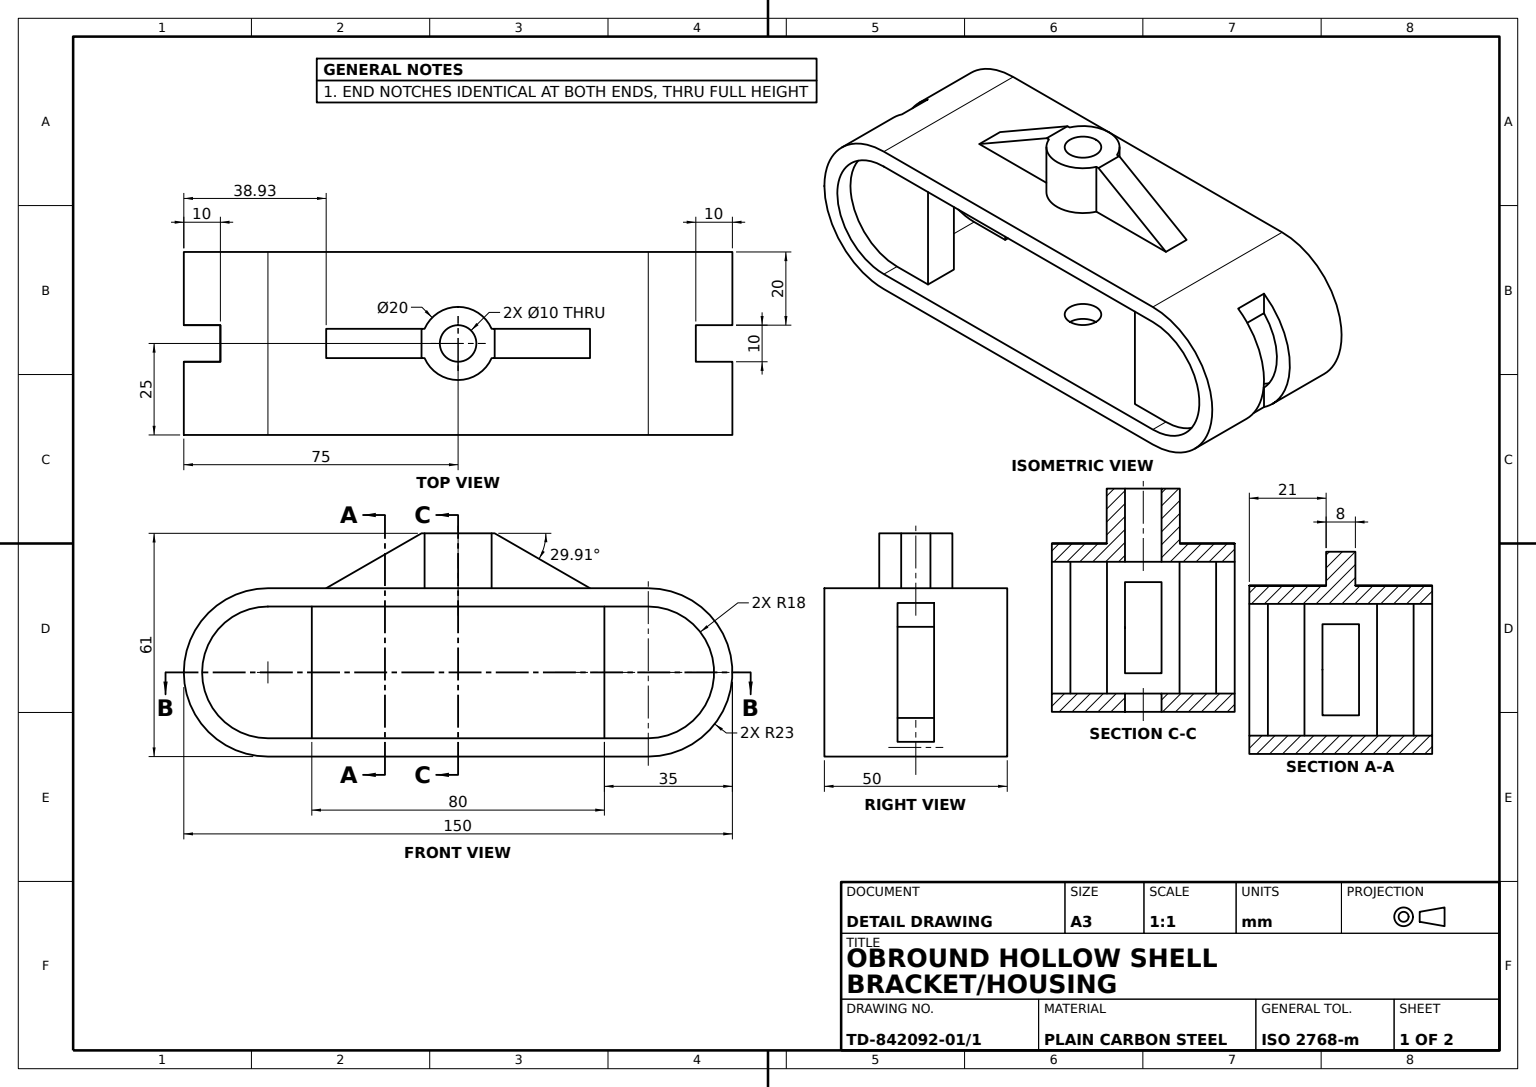
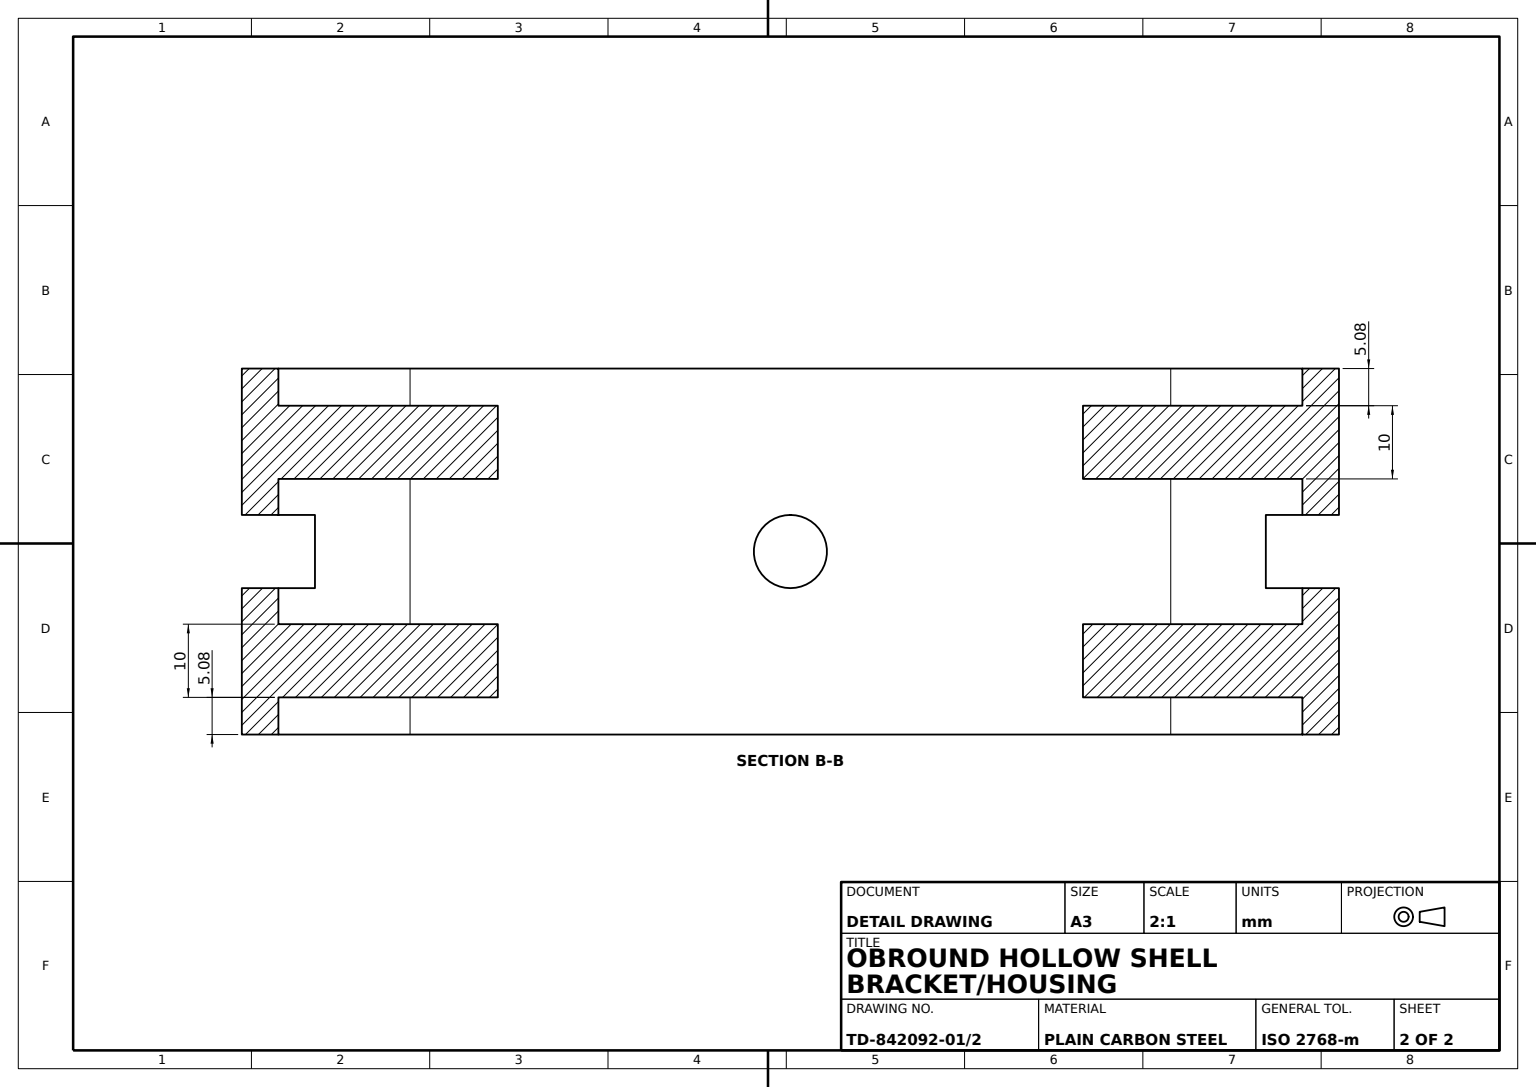
solid
v1 (-52,-18,25)
v2 (-52,-18,19.922192)
e1 v1 v2 LINE
v3 (-70,0,19.922192)
e2 v2 v3 CIRCLE(AX(P(-52,0,19.922192),D(0,0,-1),D(1,0,0)),18)
v4 (-70,0,25)
e3 v4 v3 LINE
e4 v4 v1 CIRCLE(AX(P(-52,0,25),D(0,0,1),D(1,0,0)),18)
face CYL(AX(P(-52,0,25),D(0,0,-1),D(-1,0,0)),18) rev [e1 e2 -e3 e4]
v5 (0,-23,-5)
v6 (0,-23,5)
e5 v5 v6 CIRCLE(AX(P(0,-23,0),D(0,1,0),D(0,0,1)),5)
v7 (0,-18,-5)
e6 v5 v7 LINE
v8 (0,-18,5)
e7 v7 v8 CIRCLE(AX(P(0,-18,0),D(0,1,0),D(-1,0,0)),5)
e8 v6 v8 LINE
face CYL(AX(P(0,-27,0),D(0,1,0),D(0,0,1)),5) rev [-e5 e6 e7 -e8]
v9 (40,-18,-19.922192)
v10 (40,18,-19.922192)
e9 v9 v10 LINE
v11 (40,-18,-9.922192)
e10 v11 v9 LINE
v12 (40,18,-9.922192)
e11 v11 v12 LINE
e12 v10 v12 LINE
face PLANE(AX(P(40,-23.002,-19.922192),D(-1,0,0),D(0,-1,0))) [-e9 -e10 e11 -e12]
e13 v6 v5 CIRCLE(AX(P(0,-23,0),D(0,1,0),D(0,0,1)),5)
v13 (-52,-23,25)
v14 (-52,-23,-25)
e14 v13 v14 LINE
v15 (52,-23,-25)
e15 v14 v15 LINE
v16 (52,-23,25)
e16 v16 v15 LINE
e17 v13 v16 LINE
face PLANE(AX(P(-52,-23,25),D(0,1,0),D(0,0,1))) rev [e13 e5] [e14 e15 -e16 -e17]
v17 (65,-18.973666,-5)
v18 (65,-12.4499,-5)
e18 v17 v18 LINE
v19 (65,-12.4499,5)
e19 v18 v19 LINE
v20 (65,-18.973666,5)
e20 v20 v19 LINE
e21 v17 v20 LINE
face PLANE(AX(P(65,-27,-5),D(-1,0,0),D(0,0,1))) rev [e18 e19 -e20 -e21]
v21 (-52,18,-19.922192)
v22 (-52,18,-25)
e22 v21 v22 LINE
v23 (-70,0,-19.922192)
e23 v23 v21 CIRCLE(AX(P(-52,0,-19.922192),D(0,0,-1),D(1,0,0)),18)
v24 (-70,0,-25)
e24 v23 v24 LINE
e25 v22 v24 CIRCLE(AX(P(-52,0,-25),D(0,0,1),D(1,0,0)),18)
face CYL(AX(P(-52,0,25),D(0,0,-1),D(-1,0,0)),18) rev [-e22 -e23 e24 -e25]
v25 (-10,38,4)
v26 (-36.072943,23,4)
e26 v25 v26 LINE
v27 (-9.165151,23,4)
e27 v27 v26 LINE
v28 (-9.165151,38,4)
e28 v28 v27 LINE
e29 v28 v25 LINE
face PLANE(AX(P(0,7.5,4),D(0,0,1),D(1,0,0))) [e26 -e27 -e28 e29]
v29 (-65,18.973666,-5)
v30 (-65,18.973666,5)
e30 v29 v30 LINE
v31 (-75,0,5)
e31 v30 v31 CIRCLE(AX(P(-52,0,5),D(0,0,1),D(1,0,0)),23)
v32 (-75,0,25)
e32 v32 v31 LINE
v33 (-52,23,25)
e33 v33 v32 CIRCLE(AX(P(-52,0,25),D(0,0,1),D(1,0,0)),23)
v34 (-52,23,-25)
e34 v33 v34 LINE
v35 (-75,0,-25)
e35 v34 v35 CIRCLE(AX(P(-52,0,-25),D(0,0,1),D(1,0,0)),23)
v36 (-75,0,-5)
e36 v36 v35 LINE
e37 v36 v29 CIRCLE(AX(P(-52,0,-5),D(0,0,-1),D(-1,0,0)),23)
face CYL(AX(P(-52,0,25),D(0,0,-1),D(-1,0,0)),23) [e30 e31 -e32 -e33 e34 e35 -e36 e37]
v37 (-65,12.4499,5)
v38 (-70,0,5)
e38 v37 v38 CIRCLE(AX(P(-52,0,5),D(0,0,1),D(1,0,0)),18)
v39 (-65,12.4499,-5)
e39 v39 v37 LINE
v40 (-70,0,-5)
e40 v40 v39 CIRCLE(AX(P(-52,0,-5),D(0,0,-1),D(-1,0,0)),18)
v41 (-70,0,-9.922192)
e41 v40 v41 LINE
v42 (-52,18,-9.922192)
e42 v42 v41 CIRCLE(AX(P(-52,0,-9.922192),D(0,0,1),D(-1,0,0)),18)
v43 (-52,18,9.922192)
e43 v43 v42 LINE
v44 (-70,0,9.922192)
e44 v43 v44 CIRCLE(AX(P(-52,0,9.922192),D(0,0,1),D(-1,0,0)),18)
e45 v44 v38 LINE
face CYL(AX(P(-52,0,25),D(0,0,-1),D(-1,0,0)),18) rev [-e38 -e39 -e40 e41 -e42 -e43 e44 e45]
v45 (-40,-18,-9.922192)
v46 (-40,18,-9.922192)
e46 v45 v46 LINE
e47 v46 v42 LINE
v47 (-52,-18,-9.922192)
e48 v41 v47 CIRCLE(AX(P(-52,0,-9.922192),D(0,0,1),D(-1,0,0)),18)
e49 v47 v45 LINE
face PLANE(AX(P(-40,-23.002,-9.922192),D(0,0,-1),D(-1,0,0))) rev [e46 e47 e42 e48 e49]
v48 (-52,-18,-19.922192)
e50 v48 v23 CIRCLE(AX(P(-52,0,-19.922192),D(0,0,-1),D(1,0,0)),18)
v49 (-52,-18,-25)
e51 v48 v49 LINE
e52 v24 v49 CIRCLE(AX(P(-52,0,-25),D(0,0,1),D(1,0,0)),18)
face CYL(AX(P(-52,0,25),D(0,0,-1),D(-1,0,0)),18) rev [-e24 -e50 e51 -e52]
v50 (52,23,-25)
e53 v50 v34 LINE
v51 (52,23,25)
e54 v51 v33 LINE
e55 v51 v50 LINE
v52 (36.072943,23,-4)
v53 (36.072943,23,4)
e56 v52 v53 LINE
v54 (9.165151,23,4)
e57 v53 v54 LINE
e58 v27 v54 CIRCLE(AX(P(0,23,0),D(0,1,0),D(0,0,-1)),10)
v55 (-36.072943,23,-4)
e59 v26 v55 LINE
v56 (-9.165151,23,-4)
e60 v56 v55 LINE
v57 (0,23,-10)
e61 v57 v56 CIRCLE(AX(P(0,23,0),D(0,1,0),D(0,0,-1)),10)
v58 (9.165151,23,-4)
e62 v58 v57 CIRCLE(AX(P(0,23,0),D(0,1,0),D(0,0,-1)),10)
e63 v52 v58 LINE
face PLANE(AX(P(-52,23,25),D(0,-1,0),D(0,0,-1))) rev [e53 -e34 -e54 e55] [e56 e57 -e58 e27 e59 -e60 -e61 -e62 -e63]
v59 (10,38,-4)
v60 (10,38,4)
e64 v59 v60 LINE
e65 v60 v53 LINE
e66 v59 v52 LINE
face PLANE(AX(P(10,38,0),D(-0.498672433,-0.866790519,0),D(0.866790519,-0.498672433,0))) rev [e64 e65 -e56 -e66]
v61 (-65,-12.4499,5)
v62 (-65,-12.4499,-5)
e67 v61 v62 LINE
e68 v38 v61 CIRCLE(AX(P(-52,0,5),D(0,0,1),D(1,0,0)),18)
v63 (-52,-18,9.922192)
e69 v44 v63 CIRCLE(AX(P(-52,0,9.922192),D(0,0,1),D(-1,0,0)),18)
e70 v63 v47 LINE
e71 v62 v40 CIRCLE(AX(P(-52,0,-5),D(0,0,-1),D(-1,0,0)),18)
face CYL(AX(P(-52,0,25),D(0,0,-1),D(-1,0,0)),18) rev [-e67 -e68 -e45 e69 e70 -e48 -e41 -e71]
e72 v8 v7 CIRCLE(AX(P(0,-18,0),D(0,1,0),D(-1,0,0)),5)
face CYL(AX(P(0,-27,0),D(0,1,0),D(0,0,1)),5) rev [e72 -e6 -e13 e8]
v64 (0,38,5)
v65 (0,38,-5)
e73 v64 v65 CIRCLE(AX(P(0,38,0),D(0,1,0),D(0,0,1)),5)
e74 v65 v64 CIRCLE(AX(P(0,38,0),D(0,1,0),D(0,0,1)),5)
v66 (-9.165151,38,-4)
v67 (-10,38,-4)
e75 v66 v67 LINE
e76 v67 v25 LINE
v68 (9.165151,38,4)
e77 v28 v68 CIRCLE(AX(P(0,38,0),D(0,1,0),D(0,0,1)),10)
e78 v68 v60 LINE
v69 (9.165151,38,-4)
e79 v69 v59 LINE
v70 (0,38,-10)
e80 v69 v70 CIRCLE(AX(P(0,38,0),D(0,1,0),D(0,0,1)),10)
e81 v70 v66 CIRCLE(AX(P(0,38,0),D(0,1,0),D(0,0,1)),10)
face PLANE(AX(P(0,38,0),D(0,1,0),D(0,0,1))) [-e73 -e74] [e75 e76 -e29 e77 e78 -e64 -e79 e80 e81]
v71 (40,-18,9.922192)
v72 (40,18,9.922192)
e82 v71 v72 LINE
v73 (40,-18,19.922192)
e83 v71 v73 LINE
v74 (40,18,19.922192)
e84 v73 v74 LINE
e85 v74 v72 LINE
face PLANE(AX(P(40,-23.002,19.922192),D(1,0,0),D(0,1,0))) rev [-e82 e83 e84 e85]
v75 (-40,-18,-19.922192)
e86 v75 v48 LINE
v76 (-40,18,-19.922192)
e87 v21 v76 LINE
e88 v75 v76 LINE
face PLANE(AX(P(-70,-23.002,-19.922192),D(0,0,1),D(1,0,0))) rev [e86 e50 e23 e87 -e88]
e89 v39 v29 LINE
v77 (-65,-18.973666,-5)
e90 v77 v36 CIRCLE(AX(P(-52,0,-5),D(0,0,-1),D(-1,0,0)),23)
e91 v77 v62 LINE
face PLANE(AX(P(-65,-27,-5),D(0,0,-1),D(-1,0,0))) rev [e89 -e37 -e90 e91 e71 e40]
v78 (65,18.973666,5)
e92 v20 v78 CIRCLE(AX(P(52,0,5),D(0,0,1),D(1,0,0)),23)
v79 (65,12.4499,5)
e93 v19 v79 CIRCLE(AX(P(52,0,5),D(0,0,1),D(1,0,0)),18)
e94 v79 v78 LINE
face PLANE(AX(P(65,-27,5),D(0,0,1),D(1,0,0))) rev [-e92 e20 e93 e94]
e95 v66 v56 LINE
e96 v70 v57 LINE
face CYL(AX(P(0,38,0),D(0,-1,0),D(0,0,-1)),10) [-e95 -e81 e96 e61]
e97 v67 v55 LINE
face PLANE(AX(P(-10,38,0),D(-0.498672433,0.866790519,0),D(-0.866790519,-0.498672433,0))) [-e76 e97 -e59 -e26]
v80 (52,18,9.922192)
e98 v72 v80 LINE
v81 (52,-18,9.922192)
e99 v80 v81 CIRCLE(AX(P(52,0,9.922192),D(0,0,-1),D(1,0,0)),18)
e100 v81 v71 LINE
face PLANE(AX(P(40,-23.002,9.922192),D(0,0,1),D(1,0,0))) rev [e82 e98 e99 e100]
v82 (-65,-18.973666,5)
e101 v82 v77 LINE
e102 v82 v61 LINE
face PLANE(AX(P(-65,-27,5),D(1,0,0),D(0,0,-1))) rev [-e91 -e101 e102 e67]
e103 v54 v68 LINE
face PLANE(AX(P(0,7.5,4),D(0,0,1),D(1,0,0))) [-e78 -e103 -e57 -e65]
face CYL(AX(P(0,38,0),D(0,-1,0),D(0,0,-1)),10) [e28 e58 e103 -e77]
e104 v35 v14 CIRCLE(AX(P(-52,0,-25),D(0,0,1),D(1,0,0)),23)
e105 v32 v13 CIRCLE(AX(P(-52,0,25),D(0,0,1),D(1,0,0)),23)
e106 v31 v82 CIRCLE(AX(P(-52,0,5),D(0,0,1),D(1,0,0)),23)
face CYL(AX(P(-52,0,25),D(0,0,-1),D(-1,0,0)),23) [e101 e90 e36 e104 -e14 -e105 e32 e106]
v83 (-40,-18,19.922192)
v84 (-40,18,19.922192)
e107 v83 v84 LINE
v85 (-52,18,19.922192)
e108 v85 v84 LINE
e109 v3 v85 CIRCLE(AX(P(-52,0,19.922192),D(0,0,-1),D(1,0,0)),18)
e110 v83 v2 LINE
face PLANE(AX(P(-70,-23.002,19.922192),D(0,0,1),D(1,0,0))) [e107 -e108 -e109 -e2 -e110]
v86 (52,18,-9.922192)
e111 v12 v86 LINE
e112 v80 v86 LINE
v87 (52,18,19.922192)
e113 v87 v74 LINE
v88 (52,18,25)
e114 v88 v87 LINE
v89 (-52,18,25)
e115 v88 v89 LINE
e116 v89 v85 LINE
v90 (-40,18,9.922192)
e117 v84 v90 LINE
e118 v90 v43 LINE
e119 v76 v46 LINE
v91 (52,18,-25)
e120 v91 v22 LINE
v92 (52,18,-19.922192)
e121 v92 v91 LINE
e122 v92 v10 LINE
v93 (0,18,-5)
v94 (0,18,5)
e123 v93 v94 CIRCLE(AX(P(0,18,0),D(0,-1,0),D(1,0,0)),5)
e124 v94 v93 CIRCLE(AX(P(0,18,0),D(0,-1,0),D(1,0,0)),5)
face PLANE(AX(P(-52,18,25),D(0,-1,0),D(1,0,0))) [e111 -e112 -e98 -e85 -e113 -e114 e115 e116 e108 e117 e118 e43 -e47 -e119 -e87 e22 -e120 -e121 e122 e12] [-e123 -e124]
e125 v89 v4 CIRCLE(AX(P(-52,0,25),D(0,0,1),D(1,0,0)),18)
face CYL(AX(P(-52,0,25),D(0,0,-1),D(-1,0,0)),18) rev [e3 e109 -e116 e125]
v95 (65,18.973666,-5)
e126 v95 v17 CIRCLE(AX(P(52,0,-5),D(0,0,-1),D(-1,0,0)),23)
v96 (65,12.4499,-5)
e127 v96 v95 LINE
e128 v96 v18 CIRCLE(AX(P(52,0,-5),D(0,0,-1),D(-1,0,0)),18)
face PLANE(AX(P(75,-27,-5),D(0,0,-1),D(-1,0,0))) rev [-e18 -e126 -e127 e128]
e129 v64 v94 LINE
e130 v65 v93 LINE
face CYL(AX(P(0,38,0),D(0,-1,0),D(0,0,-1)),5) rev [e74 e129 e124 -e130]
v97 (52,-18,19.922192)
e131 v73 v97 LINE
e132 v97 v87 CIRCLE(AX(P(52,0,19.922192),D(0,0,1),D(-1,0,0)),18)
face PLANE(AX(P(70,-23.002,19.922192),D(0,0,-1),D(-1,0,0))) rev [e113 -e84 e131 e132]
e133 v37 v30 LINE
face PLANE(AX(P(-65,-27,5),D(1,0,0),D(0,0,-1))) rev [-e30 -e89 e39 e133]
face CYL(AX(P(0,38,0),D(0,-1,0),D(0,0,-1)),5) rev [-e129 e73 e130 e123]
v98 (52,-18,-9.922192)
e134 v86 v98 CIRCLE(AX(P(52,0,-9.922192),D(0,0,-1),D(1,0,0)),18)
e135 v81 v98 LINE
e136 v79 v96 LINE
face CYL(AX(P(52,0,25),D(0,0,-1),D(-1,0,0)),18) rev [e134 -e135 -e99 e112] [-e93 -e19 -e128 -e136]
v99 (52,-18,-25)
e137 v49 v99 LINE
e138 v45 v75 LINE
v100 (-40,-18,9.922192)
e139 v63 v100 LINE
e140 v100 v83 LINE
v101 (52,-18,25)
e141 v1 v101 LINE
e142 v101 v97 LINE
e143 v98 v11 LINE
v102 (52,-18,-19.922192)
e144 v9 v102 LINE
e145 v102 v99 LINE
face PLANE(AX(P(-52,-18,25),D(0,1,0),D(-1,0,0))) [-e137 -e51 -e86 -e138 -e49 -e70 e139 e140 e110 -e1 e141 e142 -e131 -e83 -e100 e135 e143 e10 e144 e145] [-e72 -e7]
e146 v78 v95 LINE
e147 v15 v50 CIRCLE(AX(P(52,0,-25),D(0,0,1),D(1,0,0)),23)
e148 v16 v51 CIRCLE(AX(P(52,0,25),D(0,0,1),D(1,0,0)),23)
face CYL(AX(P(52,0,25),D(0,0,-1),D(-1,0,0)),23) [e146 e126 e21 e92] [e16 e147 -e55 -e148]
face PLANE(AX(P(40,-23.002,-9.922192),D(0,0,1),D(1,0,0))) [-e11 -e143 -e134 -e111]
e149 v101 v88 CIRCLE(AX(P(52,0,25),D(0,0,1),D(1,0,0)),18)
face PLANE(AX(P(-52,0,25),D(0,0,1),D(1,0,0))) [e105 e17 e148 e54 e33] [-e4 -e125 -e115 -e149 -e141]
e150 v100 v90 LINE
face PLANE(AX(P(-40,-23.002,19.922192),D(1,0,0),D(0,1,0))) [e150 -e117 -e107 -e140]
e151 v102 v92 CIRCLE(AX(P(52,0,-19.922192),D(0,0,1),D(-1,0,0)),18)
face PLANE(AX(P(70,-23.002,-19.922192),D(0,0,-1),D(-1,0,0))) [-e151 -e144 e9 -e122]
face PLANE(AX(P(65,-27,-5),D(-1,0,0),D(0,0,1))) rev [e127 -e146 -e94 e136]
face PLANE(AX(P(-75,-27,5),D(0,0,1),D(1,0,0))) rev [e38 e68 -e102 -e106 -e31 -e133]
e152 v99 v91 CIRCLE(AX(P(52,0,-25),D(0,0,1),D(1,0,0)),18)
face CYL(AX(P(52,0,25),D(0,0,-1),D(-1,0,0)),18) rev [-e152 -e145 e151 e121]
face PLANE(AX(P(-40,-23.002,-19.922192),D(-1,0,0),D(0,-1,0))) rev [-e46 e138 e88 e119]
e153 v58 v69 LINE
face PLANE(AX(P(0,7.5,-4),D(0,0,1),D(1,0,0))) rev [e79 e66 e63 e153]
face PLANE(AX(P(-52,0,-25),D(0,0,1),D(1,0,0))) rev [-e104 -e35 -e53 -e147 -e15] [e120 e25 e52 e137 e152]
face PLANE(AX(P(0,7.5,-4),D(0,0,1),D(1,0,0))) rev [-e75 e95 e60 -e97]
face PLANE(AX(P(-40,-23.002,9.922192),D(0,0,-1),D(-1,0,0))) [-e150 -e139 -e69 -e44 -e118]
face CYL(AX(P(52,0,25),D(0,0,-1),D(-1,0,0)),18) rev [-e142 e149 e114 -e132]
face CYL(AX(P(0,38,0),D(0,-1,0),D(0,0,-1)),10) [-e153 e62 -e96 -e80]
